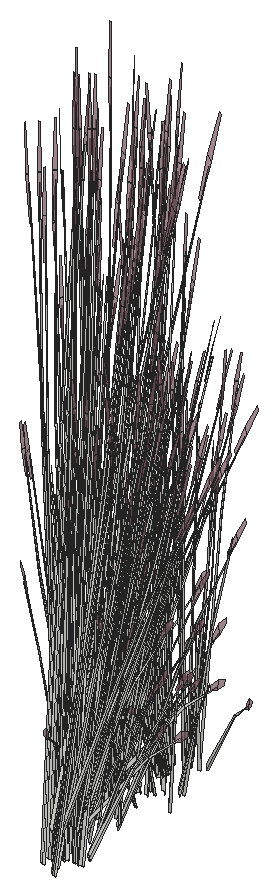
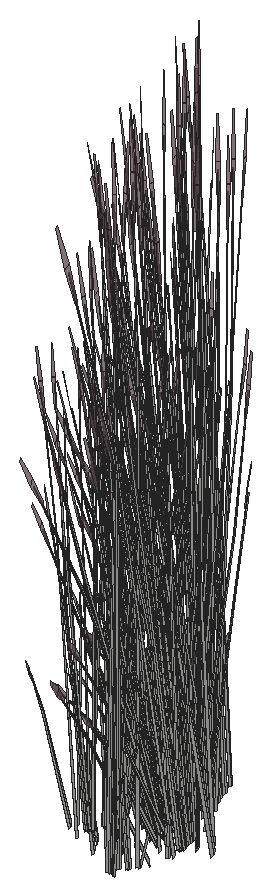
# SketchUp Ruby script. Lengths in inches.
U = 1.inch
M = Sketchup.active_model
def pt(a) = Geom::Point3d.new(a.map { |v| v * U })
def face(e, loops, mat)
  f = e.add_face(loops[0].map { |a| pt(a) })
  loops[1..].each { |l| e.add_face(l.map { |a| pt(a) }).erase! }
  f.material = f.back_material = mat if mat
  f
end
# faces: each face lists its corners as indices into pts; further lists are holes
def faces(e, pts, list, mat = nil) = list.each { |f| face(e, (f[0].is_a?(Array) ? f : [f]).map { |l| l.map { |i| pts[i] } }, mat) }
# xy, xz, yz: faces in a plane at the given z, y or x. An outline is a flat list of corners, or four numbers for a rectangle; further outlines are holes
def ring(l) = l.size == 4 ? [[l[0], l[1]], [l[2], l[1]], [l[2], l[3]], [l[0], l[3]]] : l.each_slice(2).to_a
def flat(e, list, mat, &to3) = list.each { |f| face(e, (f[0].is_a?(Array) ? f : [f]).map { |l| ring(l).map { |u, v| to3.(u, v) } }, mat) }
def xy(e, z, list, mat = nil) = flat(e, list, mat) { |x, y| [x, y, z] }
def xz(e, y, list, mat = nil) = flat(e, list, mat) { |x, z| [x, y, z] }
def yz(e, x, list, mat = nil) = flat(e, list, mat) { |y, z| [x, y, z] }
def lines(e, pts, list) = list.each { |a, b| e.add_line(pt(pts[a]), pt(pts[b])) }
# prism: a flat outline (further loops are holes) pulled along v
def prism(e, loops, v, mat = nil)
  f = face(e, loops, mat); d = Geom::Vector3d.new(v.map { |x| x * U })
  f.pushpull(f.normal.samedirection?(d) ? d.length : -d.length)
end
def box(e, o, s, mat = nil) = prism(e, [[o, [o[0] + s[0], o[1], o[2]], [o[0] + s[0], o[1] + s[1], o[2]], [o[0], o[1] + s[1], o[2]]]], [0, 0, s[2]], mat)
def at(x, y, z, deg = 0) = Geom::Transformation.translation(pt([x, y, z])) * Geom::Transformation.rotation(ORIGIN, Z_AXIS, deg.degrees)
def axes(o, x, y, z) = Geom::Transformation.new([*x, 0, *y, 0, *z, 0, *pt(o).to_a, 1])
def part(name) = M.definitions.add(name)
# library, detail: a bought-in or finely detailed component or shape, given as its bounding box
def library(name, o, s) = part(name).tap { |d| box(d.entities, o, s) }
def detail(e, o, s) = box(e.add_group.entities, o, s)
def put(e, d, t, mat = nil) = e.add_instance(d, t).tap { |i| i.material = mat if mat }
def group(e, t, mat = nil) = e.add_group.tap { |g| g.transformation = t; g.material = mat if mat }.entities
root = M.entities
M.materials.add("LightPink_Translucent").color = [144, 107, 117]
M.materials["LightPink_Translucent"].alpha = 0.75
c1 = part("blade")
p = [[2.15,0.21,22],[0,0.17,0],[0.09,0.45,0],[2.18,0.31,22],[2.29,0.31,22],[0.38,0.45,0],
  [2.48,0.24,33],[2.49,0.24,33],[2.48,0.22,33]]
faces(c1.entities,p,[[0,1,2,3],[4,5,2,3],[6,3,4,7],[8,0,3,6]])
c2 = part("seeds")
p = [[0.3,-0.1,1.38],[-0.01,-0.03,1.59],[-0.01,-0.03,0.03],[0.14,-0.07,-0.07],[0.29,-0.03,3],[0.15,0.01,3.11]]
faces(c2.entities,p,[[0,1,2,3],[1,0,4,5]],"LightPink_Translucent")
c3 = part("blade with seeds")
put(c3.entities,c1,at(0,0,0))
put(c3.entities,c2,axes([2.4,0.25,30.99],[1.5799,-0.05474,1.17369],[-0.12525,1.92788,0.29478],[-0.07173,-0.02425,1.56792]))
put(root,c3,axes([409.82,50.23,-10.12],[0.47863,0.27177,-0.46235],[-0.28609,0.48733,0],[0.10901,0.0619,1.46668]))
put(root,c3,axes([408.91,51.78,-9.95],[0.57217,0,0],[0,0.56272,0],[0,0,1.66132]))
put(root,c3,axes([406.625,56.1875,-9.59],[-0.14537,0.11002,1.33163],[-0.43536,-0.19256,-0.28638],[0.0807,-0.23948,0.56934]))
put(root,c3,axes([409.08,50.46,-9.7],[-0.54955,0.14427,0.16428],[-0.1357,-0.53689,0.32672],[0.04901,0.07823,1.49371]))
put(root,c3,axes([409.41,51.59,-8.39],[-0.21212,0.01231,1.59586],[0.14072,-0.53355,0.12904],[0.3023,0.033,0.68222]))
put(root,c3,axes([409.6875,50.43,-10.11],[0.12013,0.47362,-0.28847],[-0.47712,0.13449,0.28847],[0.09619,0.05462,1.29413]))
put(root,c3,axes([410.51,52.33,-7.6],[0.18783,0.37061,0.05988],[-0.34252,0.1814,0.47138],[0.15099,-0.03579,0.71878]))
put(root,c3,axes([408.73,51.49,-9.78],[-0.64638,-0.11452,0.45814],[0.13155,-0.64678,0.17978],[0.09446,0.06245,1.59061]))
put(root,c3,axes([410.47,52.19,-7.59],[-0.14449,0.4956,0.447],[-0.47502,-0.16947,0.36857],[0.1868,-0.02978,0.92496]))
put(root,c3,axes([408.21,53.09,-9.95],[-0.16686,-0.46861,0],[0.47648,-0.16411,0],[0,0,1.4375]))
put(root,c3,axes([406.98,57,-7.36],[0.01331,-0.50278,-0.66157],[0.56035,0.03377,0.07984],[0.05914,-0.213,0.93586]))
put(root,c3,axes([408.84,53.02,-9.97],[0.53691,-0.18442,-0.17877],[0.18866,0.53125,0.00007],[0.05927,-0.02038,1.61933]))
put(root,c3,axes([409.02,53.24,-9.7],[0.14774,-0.54019,0.16428],[0.54062,0.15287,0.32672],[-0.09339,0.00263,1.49371]))
put(root,c3,axes([407.76,56.22,-7.61],[-0.00494,-0.10818,1.62908],[-0.41695,-0.31265,-0.25764],[0.06446,-0.18952,0.13065]))
put(root,c3,axes([406.35,56.75,-8.39],[-0.09522,0.18683,1.59586],[-0.39947,-0.38663,0.12904],[0.18021,-0.24097,0.68222]))
put(root,c3,axes([408.9,52.02,-9.9375],[0.35699,0.35109,0],[-0.35699,0.35109,0],[0,0,1.57621]))
put(root,c3,axes([409.87,51.87,-9.7],[-0.40181,-0.39593,0.16428],[0.40492,-0.38402,0.32672],[-0.04438,0.08086,1.49371]))
put(root,c3,axes([409.125,51.27,-10.08],[0.53199,0.08911,-0.58063],[-0.11226,0.54969,-0.15239],[0.15876,0.06661,1.28164]))
put(root,c3,axes([411.47,52.23,-9.42],[-0.31598,0.08973,1.06958],[0.14873,-0.37085,0.78586],[0.16763,0.02538,0.23558]))
put(root,c3,axes([408.1,53.3,-9.95],[-0.51557,-0.24403,0],[0.24813,-0.50705,0],[0,0,1.51513]))
put(root,c3,axes([406.87,56.84,-7.64],[-0.3661,-0.36521,-0.47583],[0.38674,-0.31985,-0.36857],[0.0557,-0.18556,0.91046]))
put(root,c3,axes([408.9,51.61,-9.47],[0.24813,-0.48978,0.41661],[0.51557,0.23571,-0.2005],[0,0.1129,1.33761]))
put(root,c3,axes([411.33,53.8,-7.62],[-0.04624,-0.04758,1.65179],[0.10116,-0.51007,-0.15608],[0.18215,-0.03259,0.29231]))
put(root,c3,axes([408.8,51.89,-9.87],[0,0.62861,-0.05249],[-0.63949,0,0],[0,0.01975,1.67027]))
put(root,c3,axes([408.85,51.44,-9.94],[0.30722,0.45622,-0.41661],[-0.46535,0.32126,0.2005],[0.09942,0.05645,1.33761]))
put(root,c3,axes([410.93,53.37,-8.34],[-0.09788,-0.45691,-0.03251],[0.46264,-0.10504,-0.14742],[0.09661,0.02897,0.48626]))
put(root,c3,axes([409.73,53.36,-7.3125],[0.02738,-0.55277,-0.11324],[0.51847,0.01511,-0.62851],[0.19968,0.0384,0.95501]))
put(root,c3,axes([410.2,51.88,-9.69],[0,-0.54355,0.46235],[0.57217,0,0],[0,0.1238,1.46668]))
put(root,c3,axes([407.21,56.7,-7.78],[0.34603,-0.28618,-0.32977],[0.32756,0.32677,0.42575],[0.04984,-0.16603,0.81462]))
put(root,c3,axes([408.77,52.29,-9.47],[0.55535,-0.03355,0.41661],[0.05022,0.55698,-0.2005],[-0.09942,0.05645,1.33761]))
put(root,c3,axes([409.11,51.72,-9.5625],[0.47648,-0.15851,0.13483],[0.16686,0.45265,-0.38503],[0,0.09962,1.18024]))
put(root,c3,axes([409.65,53.14,-7.3],[-0.29098,-0.34031,0.32977],[0.33226,-0.32215,-0.42575],[0.16881,0.04902,0.81462]))
put(root,c3,axes([410.88,52.82,-9.59],[-0.12317,-0.13368,1.33163],[0.16025,-0.44223,-0.28638],[0.24919,0.05991,0.56934]))
put(root,c3,axes([408.68,53.31,-9.95],[0.51557,0.24403,0],[-0.24813,0.50705,0],[0,0,1.62917]))
put(root,c3,axes([410.18,53.03,-7.61],[0.10971,-0.00919,1.62908],[0.30091,-0.42228,-0.25764],[0.19514,0.05574,0.13065]))
put(root,c3,axes([408.77,52.53,-9.5625],[0.37783,0.32657,0.13483],[-0.31516,0.36844,-0.38503],[-0.08772,0.04981,1.18024]))
put(root,c3,axes([407.64,56.53,-10.61],[-0.07655,-0.04282,1.6421],[-0.19662,-0.47839,-0.25086],[0.13264,-0.12982,0.2797]))
put(root,c3,axes([407.21,56.8125,-7.59],[0.36417,0.37086,0.447],[-0.38674,0.31985,0.36857],[0.06718,-0.174,0.92496]))
put(root,c3,axes([409.75,53.09,-7.36],[0.51122,0.01309,-0.66157],[-0.03434,0.5511,0.07984],[0.21658,0.05816,0.93586]))
put(root,c3,axes([407.34,56.85,-7.6],[0.42027,0.02533,0.05988],[-0.01152,0.38243,0.47138],[0.04398,-0.14649,0.71878]))
put(root,c3,axes([409.18,53.53,-9.69],[0.47863,-0.27177,0.46235],[0.28609,0.48733,0],[-0.10901,0.0619,1.46668]))
put(root,c3,axes([407.03,57.11,-7.3],[-0.34603,0.28618,0.32977],[-0.32756,-0.32677,-0.42575],[0.04984,-0.16603,0.81462]))
put(root,c3,axes([408.5,53.11,-9.87],[0.22235,0.62444,-0.05599],[-0.63531,0.21881,0],[0.00776,0.02181,1.60327]))
put(root,c3,axes([407.64,57.875,-7.36],[0.26714,-0.42887,-0.66157],[0.46811,0.30479,0.07984],[0.1595,-0.15539,0.93586]))
put(root,c3,axes([407.625,57.68,-7.64],[-0.13138,-0.49631,-0.47583],[0.49754,-0.08682,-0.36857],[0.14258,-0.13331,0.91046]))
put(root,c3,axes([410.59,51.97,-9.79],[0.63949,0,0],[0,0.60749,-0.48057],[0,0.13836,1.52448]))
put(root,c3,axes([410.33,52.29,-9.95],[-0.63917,-0.00435,-0.04634],[0,-0.60749,0.46507],[-0.02009,0.13829,1.47457]))
put(root,c3,axes([408.95,51.76,-9.52],[0.57594,0.25935,-0.27094],[-0.27732,0.5474,-0.46562],[0.0181,0.1344,1.4872]))
put(root,c3,axes([410.06,53.32,-7.78],[0.29098,0.34031,-0.32977],[-0.33226,0.32215,0.42575],[0.16881,0.04902,0.81462]))
put(root,c3,axes([410.2,52.375,-10.11],[-0.35699,0.33913,-0.28847],[-0.35699,-0.33913,0.28847],[0,0.10923,1.29413]))
put(root,c3,axes([407.86,58.03,-7.3125],[-0.47307,-0.29971,-0.11324],[0.27254,-0.43404,-0.62851],[0.13365,-0.15087,0.95501]))
put(root,c3,axes([409.91,53.45,-7.6],[-0.02575,0.41332,0.05988],[-0.38885,-0.01133,0.47138],[0.14895,0.04325,0.71878]))
put(root,c3,axes([408.89,52.16,-9.94],[-0.24813,0.48978,-0.41661],[-0.51557,-0.23571,0.2005],[0,0.1129,1.33761]))
put(root,c3,axes([409.95,53.32,-7.59],[-0.37709,0.35815,0.447],[-0.32522,-0.38035,0.36857],[0.17692,0.06607,0.92496]))
put(root,c3,axes([405.1875,56.54,-10.12],[0.47863,-0.27177,-0.46235],[0.28609,0.48733,0],[0.10901,-0.0619,1.46668]))
put(root,c3,axes([408.03,57.48,-9.59],[-0.1827,-0.0161,1.33163],[-0.18717,-0.43188,-0.28638],[0.22444,-0.12218,0.56934]))
put(root,c3,axes([409.03,57.9,-7.62],[-0.0668,-0.00413,1.65179],[-0.27738,-0.44233,-0.15608],[0.11139,-0.14544,0.29231]))
put(root,c3,axes([405.75,57.66,-10.08],[0.34446,-0.40855,-0.58063],[0.42791,0.37046,-0.15239],[0.13803,-0.10191,1.28164]))
put(root,c3,axes([408.24,56.6875,-9.42],[-0.17034,0.27669,1.06958],[-0.14642,-0.37174,0.78586],[0.14069,-0.09315,0.23558]))
put(root,c3,axes([408.75,53.73,-7.3],[-0.07899,-0.43781,0.32977],[0.45153,-0.11561,-0.42575],[0.12128,0.12546,0.81462]))
put(root,c3,axes([408.9,53.57,-9.83],[0.64025,0.17667,0.2864],[-0.16018,0.63149,-0.33981],[-0.10597,0.07904,1.53541]))
put(root,c3,axes([410.44,52.39,-10.12],[0,0.54355,-0.46235],[-0.57217,0,0],[0,0.1238,1.46668]))
put(root,c3,axes([409.01,52.45,-8.39],[-0.18996,-0.09365,1.59586],[0.39312,-0.39287,0.12904],[0.24502,0.17723,0.68222]))
put(root,c3,axes([409.05,51.21,-7.83],[-0.44191,-0.28242,1.28769],[0.46662,-0.43971,0.5556],[0.14258,0.26499,1.24467]))
put(root,c3,axes([407.99,57.73,-7.78],[0.44516,-0.07768,-0.32977],[0.11755,0.44407,0.42575],[0.12757,-0.11927,0.81462]))
put(root,c3,axes([409.72,53.51,-9.42],[-0.28795,-0.15629,1.06958],[0.37181,-0.1588,0.78586],[0.10029,0.13452,0.23558]))
put(root,c3,axes([408.71,53.96,-7.3125],[0.30474,-0.46525,-0.11324],[0.44133,0.26804,-0.62851],[0.15341,0.13145,0.95501]))
put(root,c3,axes([405.38,58.13,-9.52],[-0.05959,-0.62022,-0.27094],[0.62068,-0.0375,-0.46562],[0.1093,-0.08261,1.4872]))
put(root,c3,axes([407.63,57.99,-7.3],[-0.44516,0.07768,0.32977],[-0.11755,-0.44407,-0.42575],[0.12757,-0.11927,0.81462]))
put(root,c3,axes([409.29,53.91,-9.79],[0.31974,0.54466,0],[-0.53494,0.30375,-0.48057],[-0.12184,0.06918,1.52448]))
put(root,c3,axes([405.3,56.76,-10.11],[0.47712,0.13449,-0.28847],[-0.12013,0.47362,0.28847],[0.09619,-0.05462,1.29413]))
put(root,c3,axes([408.31,54.35,-7.62],[0.00151,-0.06581,1.65179],[0.43826,-0.29033,-0.15608],[0.15223,0.10363,0.29231]))
put(root,c3,axes([409.8,54.09,-10.61],[0.03726,-0.07847,1.6421],[0.46909,-0.23111,-0.25086],[0.14221,0.11962,0.2797]))
put(root,c3,axes([409.18,52.3125,-10.05],[0.18752,0.49766,-0.6445],[-0.54017,0.17923,-0.16915],[0.02073,0.16852,1.42262]))
put(root,c3,axes([409.07,53.73,-7.64],[0.50465,-0.12921,-0.47583],[0.08828,0.48932,-0.36857],[0.13555,0.14022,0.91046]))
put(root,c3,axes([407.67,53.8,-7.3],[0.15418,-0.41799,0.32977],[0.44981,0.12192,-0.42575],[0.04124,0.16829,0.81462]))
put(root,c3,axes([408.03,57.92,-7.6],[0.35109,0.22859,0.05988],[-0.2044,0.32553,0.47138],[0.11256,-0.10524,0.71878]))
put(root,c3,axes([407.9375,57.82,-7.59],[0.12683,0.50025,0.447],[-0.49754,0.08682,0.36857],[0.14663,-0.11765,0.92496]))
put(root,c3,axes([409.76,54.23,-9.52],[-0.32795,-0.01705,0.97832],[0.21658,-0.36206,0.54015],[0.12956,0.12863,0.76741]))
put(root,c3,axes([409.28,58.43,-7.61],[0.07097,-0.08279,1.62908],[-0.09083,-0.50786,-0.25764],[0.17806,-0.09629,0.13065]))
put(root,c3,axes([408.82,54.13,-7.6],[-0.23243,0.34529,0.05988],[-0.331,-0.20103,0.47138],[0.10701,0.1107,0.71878]))
put(root,c3,axes([408.27,55.29,-6.74],[0.35341,-0.31182,-0.06041],[0.32382,0.34152,-0.27392],[0.0228,0.09677,0.90349]))
put(root,c3,axes([408.92,54.03,-7.59],[-0.50866,0.12474,0.447],[-0.08828,-0.48932,0.36857],[0.11963,0.14421,0.92496]))
put(root,c3,axes([408.69,53.35,-9.59],[0.00902,-0.18018,1.33163],[0.43127,-0.20126,-0.28638],[0.13313,0.21566,0.56934]))
put(root,c3,axes([407.53,54.18,-7.6],[-0.37684,0.18473,0.05988],[-0.18445,-0.33686,0.47138],[0.03639,0.14849,0.71878]))
put(root,c3,axes([407.52,53.98,-7.3125],[0.50045,-0.25306,-0.11324],[0.24593,0.44915,-0.62851],[0.06603,0.18927,0.95501]))
put(root,c3,axes([407.66,54.15,-7.28],[-0.50393,-0.1421,0.49617],[0.17232,-0.46717,0.40911],[0.03028,0.18372,1.0267]))
put(root,c3,axes([407.88,59.2,-7.3125],[-0.25732,-0.49218,-0.11324],[0.45669,-0.24187,-0.62851],[0.19245,-0.06494,0.95501]))
put(root,c3,axes([407.86,58.78,-7.64],[0.13855,-0.49442,-0.47583],[0.47502,0.16947,-0.36857],[0.19125,-0.04534,0.91046]))
put(root,c3,axes([407.11,56.77,-9.79],[0.31974,-0.54466,0],[0.53494,0.30375,-0.48057],[0.12184,0.06918,1.52448]))
put(root,c3,axes([407.61,54.08,-10.61],[0.08277,-0.02958,1.6421],[0.49786,0.16279,-0.25086],[0.01456,0.18348,0.2797]))
put(root,c3,axes([408.37,58.92,-10.15],[-0.32938,0.06523,1.31842],[-0.05243,-0.51922,0.07547],[0.2307,-0.07859,0.75023]))
put(root,c3,axes([408.97,58.46,-9.89],[-0.31706,-0.34757,-0.06041],[0.34725,-0.31847,-0.27392],[0.09839,-0.02242,0.90349]))
put(root,c3,axes([407.95,53.96,-7.64],[0.50273,0.13626,-0.47583],[-0.17232,0.46717,-0.36857],[0.0461,0.18809,0.91046]))
put(root,c3,axes([408.23,52.99,-8.39],[-0.1169,-0.17452,1.59586],[0.54019,-0.14692,0.12904],[0.12209,0.27397,0.68222]))
put(root,c3,axes([406.83,57.05,-9.69],[-0.47863,-0.27177,0.46235],[0.28609,-0.48733,0],[0.10901,0.0619,1.46668]))
put(root,c3,axes([407.77,58.96,-7.36],[0.44939,-0.24006,-0.66157],[0.25044,0.49415,0.07984],[0.21713,-0.05613,0.93586]))
put(root,c3,axes([407.72,54.24,-7.78],[-0.15418,0.41799,-0.32977],[-0.44981,-0.12192,0.42575],[0.04124,0.16829,0.81462]))
put(root,c3,axes([409.0625,62.16,-9.59],[-0.14537,0.11002,1.33163],[-0.43536,-0.19256,-0.28638],[0.0807,-0.23948,0.56934]))
put(root,c3,axes([407.7,59.05,-7.3],[-0.42502,-0.15163,0.32977],[0.12396,-0.44238,-0.42575],[0.17112,-0.04056,0.81462]))
put(root,c3,axes([404.79,57.73,-10.52],[-0.50338,0.21762,1.20058],[-0.16022,-0.62439,0.4665],[0.30911,0.01039,1.36553]))
put(root,c3,axes([406.15,57.89,-9.5625],[0.09866,-0.48509,0.13483],[0.48202,0.0842,-0.38503],[0.08772,0.04981,1.18024]))
put(root,c3,axes([407.98,61.57,-10.61],[-0.08578,0.01958,1.6421],[-0.47437,-0.22044,-0.25086],[0.00796,-0.18387,0.2797]))
put(root,c3,axes([408.72,58.58,-10.61],[-0.02673,-0.08252,1.6421],[0.18538,-0.48271,-0.25086],[0.187,-0.00694,0.2797]))
put(root,c3,axes([405.9375,58.02,-9.47],[-0.30722,-0.45622,0.41661],[0.46535,-0.32126,-0.2005],[0.09942,0.05645,1.33761]))
put(root,c3,axes([409.41,62.98,-7.36],[0.01331,-0.50278,-0.66157],[0.56035,0.03377,0.07984],[0.05914,-0.213,0.93586]))
put(root,c3,axes([407.76,53.87,-7.36],[0.24409,0.44196,-0.66157],[-0.50245,0.2463,0.07984],[0.05708,0.21354,0.93586]))
put(root,c3,axes([410.2,62.19,-7.61],[-0.00494,-0.10818,1.62908],[-0.41695,-0.31265,-0.25764],[0.06446,-0.18952,0.13065]))
put(root,c3,axes([408.44,62.17,-7.78],[0.15418,-0.41799,-0.32977],[0.44981,0.12192,0.42575],[-0.04124,-0.16829,0.81462]))
put(root,c3,axes([408.78,62.72,-8.39],[-0.09522,0.18683,1.59586],[-0.39947,-0.38663,0.12904],[0.18021,-0.24097,0.68222]))
put(root,c3,axes([410.08,61.8,-7.62],[-0.05194,0.04152,1.65179],[-0.50886,-0.14007,-0.15608],[-0.01842,-0.18118,0.29231]))
put(root,c3,axes([406.1,58.05,-9.52],[0.51635,-0.36087,-0.27094],[0.34336,0.5099,-0.46562],[0.1274,0.05178,1.4872]))
put(root,c3,axes([408.15,59,-7.78],[0.42502,0.15163,-0.32977],[-0.12396,0.44238,0.42575],[0.17112,-0.04056,0.81462]))
put(root,c3,axes([407.4,54.98,-7.61],[0.06483,0.08753,1.62908],[0.52315,0.03439,-0.25764],[0.05261,0.19303,0.13065]))
put(root,c3,axes([407.4,57.09,-10.12],[0.47863,0.27177,-0.46235],[-0.28609,0.48733,0],[0.10901,0.0619,1.46668]))
put(root,c3,axes([406.49,58.64,-9.95],[0.57217,0,0],[0,0.56272,0],[0,0,1.66132]))
put(root,c3,axes([408.53,61.29,-9.42],[0.06561,0.31695,1.06958],[-0.36394,-0.17555,0.78586],[0.03916,-0.16229,0.23558]))
put(root,c3,axes([409.3,62.8125,-7.64],[-0.3661,-0.36521,-0.47583],[0.38674,-0.31985,-0.36857],[0.0557,-0.18556,0.91046]))
put(root,c3,axes([406.99,58.46,-8.39],[-0.21212,0.01231,1.59586],[0.14072,-0.53355,0.12904],[0.3023,0.033,0.68222]))
put(root,c3,axes([407.26,57.3,-10.11],[0.12013,0.47362,-0.28847],[-0.47712,0.13449,0.28847],[0.09619,0.05462,1.29413]))
put(root,c3,axes([408.09,59.19,-7.6],[0.18783,0.37061,0.05988],[-0.34252,0.1814,0.47138],[0.15099,-0.03579,0.71878]))
put(root,c3,axes([408.05,59.06,-7.59],[-0.14449,0.4956,0.447],[-0.47502,-0.16947,0.36857],[0.1868,-0.02978,0.92496]))
put(root,c3,axes([408.5,62.27,-7.59],[0.50393,0.1421,0.447],[-0.17232,0.46717,0.36857],[-0.03028,-0.18372,0.92496]))
put(root,c3,axes([409.68,63,-7.3125],[-0.56206,-0.02693,-0.11324],[0.01536,-0.50991,-0.62851],[0.03904,-0.19638,0.95501]))
put(root,c3,axes([409.65,62.68,-7.78],[0.34603,-0.28618,-0.32977],[0.32756,0.32677,0.42575],[0.04984,-0.16603,0.81462]))
put(root,c3,axes([408.63,62.23,-7.6],[0.37684,-0.18473,0.05988],[0.18445,0.33686,0.47138],[-0.03639,-0.14849,0.71878]))
put(root,c3,axes([406.41,59.89,-9.97],[0.53691,-0.18442,-0.17877],[0.18866,0.53125,0.00007],[0.05927,-0.02038,1.61933]))
put(root,c3,axes([406.7,58.13,-10.08],[0.53199,0.08911,-0.58063],[-0.11226,0.54969,-0.15239],[0.15876,0.06661,1.28164]))
put(root,c3,axes([409.05,59.09,-9.42],[-0.31598,0.08973,1.06958],[0.14873,-0.37085,0.78586],[0.16763,0.02538,0.23558]))
put(root,c3,axes([408.9,60.66,-7.62],[-0.04624,-0.04758,1.65179],[0.10116,-0.51007,-0.15608],[0.18215,-0.03259,0.29231]))
put(root,c3,axes([410.08,62.5,-10.61],[-0.07655,-0.04282,1.6421],[-0.19662,-0.47839,-0.25086],[0.13264,-0.12982,0.2797]))
put(root,c3,axes([406.42,58.31,-9.94],[0.30722,0.45622,-0.41661],[-0.46535,0.32126,0.2005],[0.09942,0.05645,1.33761]))
put(root,c3,axes([408.5,60.24,-8.34],[-0.09788,-0.45691,-0.03251],[0.46264,-0.10504,-0.14742],[0.09661,0.02897,0.48626]))
put(root,c3,axes([407.3,60.22,-7.3125],[0.02738,-0.55277,-0.11324],[0.51847,0.01511,-0.62851],[0.19968,0.0384,0.95501]))
put(root,c3,axes([408.49,62.61,-7.3],[-0.15418,0.41799,0.32977],[-0.44981,-0.12192,-0.42575],[-0.04124,-0.16829,0.81462]))
put(root,c3,axes([407.77,58.75,-9.69],[0,-0.54355,0.46235],[0.57217,0,0],[0,0.1238,1.46668]))
put(root,c3,axes([409.64,62.79,-7.59],[0.36417,0.37086,0.447],[-0.38674,0.31985,0.36857],[0.06718,-0.174,0.92496]))
put(root,c3,axes([406.6875,58.59,-9.5625],[0.47648,-0.15851,0.13483],[0.16686,0.45265,-0.38503],[0,0.09962,1.18024]))
put(root,c3,axes([409.78,62.82,-7.6],[0.42027,0.02533,0.05988],[-0.01152,0.38243,0.47138],[0.04398,-0.14649,0.71878]))
put(root,c3,axes([407.22,60.01,-7.3],[-0.29098,-0.34031,0.32977],[0.33226,-0.32215,-0.42575],[0.16881,0.04902,0.81462]))
put(root,c3,axes([409.46,63.08,-7.3],[-0.34603,0.28618,0.32977],[-0.32756,-0.32677,-0.42575],[0.04984,-0.16603,0.81462]))
put(root,c3,axes([410.07,63.85,-7.36],[0.26714,-0.42887,-0.66157],[0.46811,0.30479,0.07984],[0.1595,-0.15539,0.93586]))
put(root,c3,axes([408.46,59.6875,-9.59],[-0.12317,-0.13368,1.33163],[0.16025,-0.44223,-0.28638],[0.24919,0.05991,0.56934]))
put(root,c3,axes([407.1875,62.6,-9.79],[-0.31974,-0.54466,0],[0.53494,-0.30375,-0.48057],[0.12184,-0.06918,1.52448]))
put(root,c3,axes([410.0625,63.65,-7.64],[-0.13138,-0.49631,-0.47583],[0.49754,-0.08682,-0.36857],[0.14258,-0.13331,0.91046]))
put(root,c3,axes([410.3,64.01,-7.3125],[-0.47307,-0.29971,-0.11324],[0.27254,-0.43404,-0.62851],[0.13365,-0.15087,0.95501]))
put(root,c3,axes([407.75,59.89,-7.61],[0.10971,-0.00919,1.62908],[0.30091,-0.42228,-0.25764],[0.19514,0.05574,0.13065]))
put(root,c3,axes([407.62,62.52,-10.12],[0.47863,-0.27177,-0.46235],[0.28609,0.48733,0],[0.10901,-0.0619,1.46668]))
put(root,c3,axes([410.46,63.46,-9.59],[-0.1827,-0.0161,1.33163],[-0.18717,-0.43188,-0.28638],[0.22444,-0.12218,0.56934]))
put(root,c3,axes([407.33,59.96,-7.36],[0.51122,0.01309,-0.66157],[-0.03434,0.5511,0.07984],[0.21658,0.05816,0.93586]))
put(root,c3,axes([411.46,63.88,-7.62],[-0.0668,-0.00413,1.65179],[-0.27738,-0.44233,-0.15608],[0.11139,-0.14544,0.29231]))
put(root,c3,axes([408.1875,63.63,-10.08],[0.34446,-0.40855,-0.58063],[0.42791,0.37046,-0.15239],[0.13803,-0.10191,1.28164]))
put(root,c3,axes([410.67,62.66,-9.42],[-0.17034,0.27669,1.06958],[-0.14642,-0.37174,0.78586],[0.14069,-0.09315,0.23558]))
put(root,c3,axes([408.16,58.84,-9.79],[0.63949,0,0],[0,0.60749,-0.48057],[0,0.13836,1.52448]))
put(root,c3,axes([410.43,63.7,-7.78],[0.44516,-0.07768,-0.32977],[0.11755,0.44407,0.42575],[0.12757,-0.11927,0.81462]))
put(root,c3,axes([406.52,58.62,-9.52],[0.57594,0.25935,-0.27094],[-0.27732,0.5474,-0.46562],[0.0181,0.1344,1.4872]))
put(root,c3,axes([407.64,60.18,-7.78],[0.29098,0.34031,-0.32977],[-0.33226,0.32215,0.42575],[0.16881,0.04902,0.81462]))
put(root,c3,axes([407.59,64.35,-9.94],[0.24813,-0.48978,-0.41661],[0.51557,0.23571,0.2005],[0,-0.1129,1.33761]))
put(root,c3,axes([407.49,60.32,-7.6],[-0.02575,0.41332,0.05988],[-0.38885,-0.01133,0.47138],[0.14895,0.04325,0.71878]))
put(root,c3,axes([407.81,64.11,-9.52],[-0.05959,-0.62022,-0.27094],[0.62068,-0.0375,-0.46562],[0.1093,-0.08261,1.4872]))
put(root,c3,axes([407.52,60.18,-7.59],[-0.37709,0.35815,0.447],[-0.32522,-0.38035,0.36857],[0.17692,0.06607,0.92496]))
put(root,c3,axes([410.07,63.97,-7.3],[-0.44516,0.07768,0.32977],[-0.11755,-0.44407,-0.42575],[0.12757,-0.11927,0.81462]))
put(root,c3,axes([407.73,62.73,-10.11],[0.47712,0.13449,-0.28847],[-0.12013,0.47362,0.28847],[0.09619,-0.05462,1.29413]))
put(root,c3,axes([406.32,60.6,-7.3],[-0.07899,-0.43781,0.32977],[0.45153,-0.11561,-0.42575],[0.12128,0.12546,0.81462]))
put(root,c3,axes([408.02,59.25,-10.12],[0,0.54355,-0.46235],[-0.57217,0,0],[0,0.1238,1.46668]))
put(root,c3,axes([406.59,59.3125,-8.39],[-0.18996,-0.09365,1.59586],[0.39312,-0.39287,0.12904],[0.24502,0.17723,0.68222]))
put(root,c3,axes([406.625,58.08,-7.83],[-0.44191,-0.28242,1.28769],[0.46662,-0.43971,0.5556],[0.14258,0.26499,1.24467]))
put(root,c3,axes([410.47,63.9,-7.6],[0.35109,0.22859,0.05988],[-0.2044,0.32553,0.47138],[0.11256,-0.10524,0.71878]))
put(root,c3,axes([410.37,63.8,-7.59],[0.12683,0.50025,0.447],[-0.49754,0.08682,0.36857],[0.14663,-0.11765,0.92496]))
put(root,c3,axes([411.71,64.41,-7.61],[0.07097,-0.08279,1.62908],[-0.09083,-0.50786,-0.25764],[0.17806,-0.09629,0.13065]))
put(root,c3,axes([407.29,60.38,-9.42],[-0.28795,-0.15629,1.06958],[0.37181,-0.1588,0.78586],[0.10029,0.13452,0.23558]))
put(root,c3,axes([406.28,60.82,-7.3125],[0.30474,-0.46525,-0.11324],[0.44133,0.26804,-0.62851],[0.15341,0.13145,0.95501]))
put(root,c3,axes([407.9,64.59,-9.73],[0.57623,0.26344,0.22409],[-0.27732,0.5474,0.46562],[0,-0.12618,1.49497]))
put(root,c3,axes([405.88,61.21,-7.62],[0.00151,-0.06581,1.65179],[0.43826,-0.29033,-0.15608],[0.15223,0.10363,0.29231]))
put(root,c3,axes([407.375,60.96,-10.61],[0.03726,-0.07847,1.6421],[0.46909,-0.23111,-0.25086],[0.14221,0.11962,0.2797]))
put(root,c3,axes([406.75,59.18,-10.05],[0.18752,0.49766,-0.6445],[-0.54017,0.17923,-0.16915],[0.02073,0.16852,1.42262]))
put(root,c3,axes([406.64,60.59,-7.64],[0.50465,-0.12921,-0.47583],[0.08828,0.48932,-0.36857],[0.13555,0.14022,0.91046]))
put(root,c3,axes([407.71,64.23,-9.47],[-0.55535,0.03355,0.41661],[-0.05022,-0.55698,-0.2005],[0.09942,-0.05645,1.33761]))
put(root,c3,axes([410.32,65.18,-7.3125],[-0.25732,-0.49218,-0.11324],[0.45669,-0.24187,-0.62851],[0.19245,-0.06494,0.95501]))
